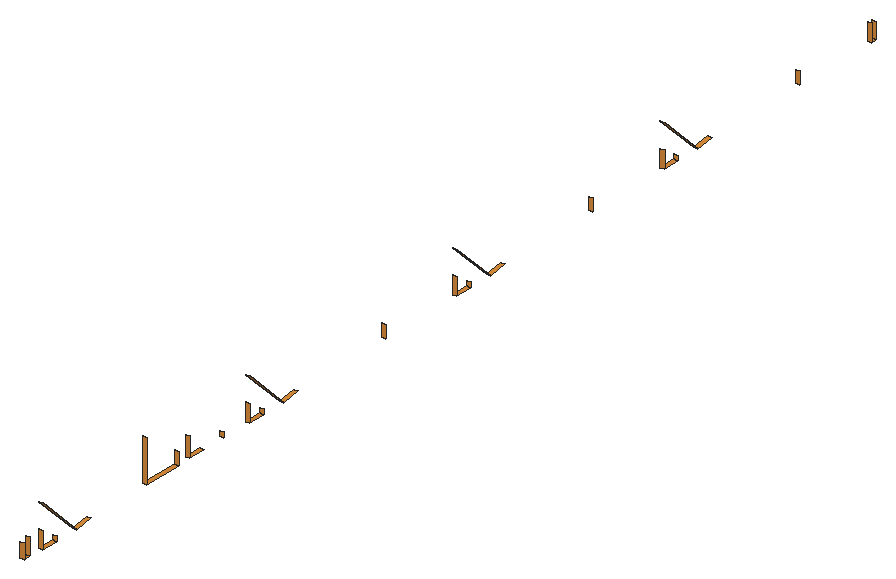
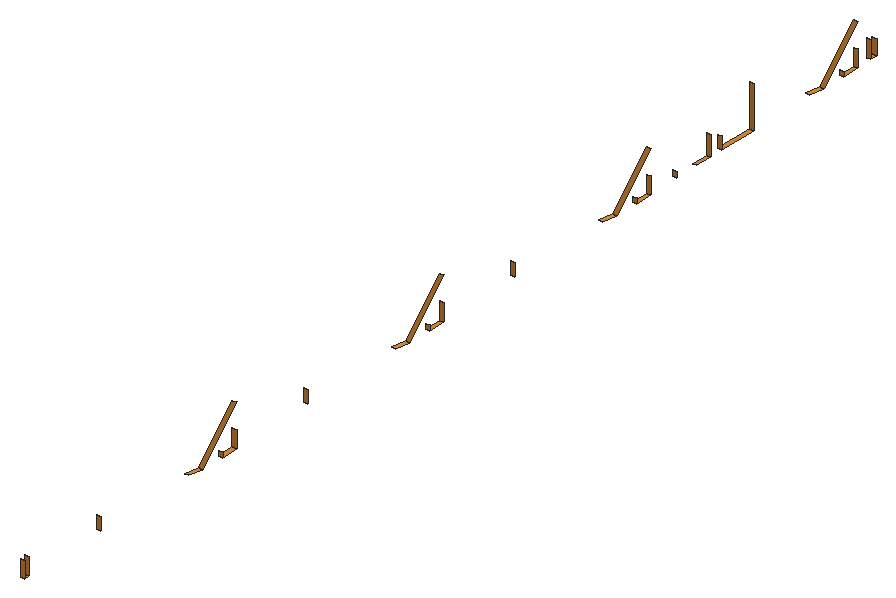
# SketchUp Ruby script. Lengths in inches.
U = 1.inch
M = Sketchup.active_model
def pt(a) = Geom::Point3d.new(a.map { |v| v * U })
def face(e, loops, mat)
  f = e.add_face(loops[0].map { |a| pt(a) })
  loops[1..].each { |l| e.add_face(l.map { |a| pt(a) }).erase! }
  f.material = f.back_material = mat if mat
  f
end
# faces: each face lists its corners as indices into pts; further lists are holes
def faces(e, pts, list, mat = nil) = list.each { |f| face(e, (f[0].is_a?(Array) ? f : [f]).map { |l| l.map { |i| pts[i] } }, mat) }
# xy, xz, yz: faces in a plane at the given z, y or x. An outline is a flat list of corners, or four numbers for a rectangle; further outlines are holes
def ring(l) = l.size == 4 ? [[l[0], l[1]], [l[2], l[1]], [l[2], l[3]], [l[0], l[3]]] : l.each_slice(2).to_a
def flat(e, list, mat, &to3) = list.each { |f| face(e, (f[0].is_a?(Array) ? f : [f]).map { |l| ring(l).map { |u, v| to3.(u, v) } }, mat) }
def xy(e, z, list, mat = nil) = flat(e, list, mat) { |x, y| [x, y, z] }
def xz(e, y, list, mat = nil) = flat(e, list, mat) { |x, z| [x, y, z] }
def yz(e, x, list, mat = nil) = flat(e, list, mat) { |y, z| [x, y, z] }
def lines(e, pts, list) = list.each { |a, b| e.add_line(pt(pts[a]), pt(pts[b])) }
# prism: a flat outline (further loops are holes) pulled along v
def prism(e, loops, v, mat = nil)
  f = face(e, loops, mat); d = Geom::Vector3d.new(v.map { |x| x * U })
  f.pushpull(f.normal.samedirection?(d) ? d.length : -d.length)
end
def box(e, o, s, mat = nil) = prism(e, [[o, [o[0] + s[0], o[1], o[2]], [o[0] + s[0], o[1] + s[1], o[2]], [o[0], o[1] + s[1], o[2]]]], [0, 0, s[2]], mat)
def at(x, y, z, deg = 0) = Geom::Transformation.translation(pt([x, y, z])) * Geom::Transformation.rotation(ORIGIN, Z_AXIS, deg.degrees)
def axes(o, x, y, z) = Geom::Transformation.new([*x, 0, *y, 0, *z, 0, *pt(o).to_a, 1])
def part(name) = M.definitions.add(name)
# library, detail: a bought-in or finely detailed component or shape, given as its bounding box
def library(name, o, s) = part(name).tap { |d| box(d.entities, o, s) }
def detail(e, o, s) = box(e.add_group.entities, o, s)
def put(e, d, t, mat = nil) = e.add_instance(d, t).tap { |i| i.material = mat if mat }
def group(e, t, mat = nil) = e.add_group.tap { |g| g.transformation = t; g.material = mat if mat }.entities
root = M.entities
M.materials.add("1056 AP 9903 Mellow Melon-N").color = [219, 142, 59]
xy(root,148.04,[[14.35,18.88,15.0625,21.91],[14.35,64.22,15.0625,67.26],[14.35,109.57,15.0625,112.6],[14.35,154.91,15.0625,157.94],[14.35,200.25,15.0625,201.3125]],"1056 AP 9903 Mellow Melon-N")
xy(root,148.27,[[14.35,14.79,15.0625,16.07],[14.35,41.65,15.0625,48.53],[14.35,51.11,15.0625,54.08]],"1056 AP 9903 Mellow Melon-N")
xz(root,14.79,[[14.35,148.27,15.0625,150.86]],"1056 AP 9903 Mellow Melon-N")
xz(root,16.07,[[14.35,148.27,15.0625,151.3]],"1056 AP 9903 Mellow Melon-N")
xz(root,18.88,[[14.35,148.04,15.0625,151.05]],"1056 AP 9903 Mellow Melon-N")
xz(root,21.91,[[14.35,148.04,15.0625,148.89]],"1056 AP 9903 Mellow Melon-N")
xz(root,41.65,[[14.35,148.27,15.0625,155.63]],"1056 AP 9903 Mellow Melon-N")
xz(root,48.53,[[14.35,148.27,15.0625,150.43]],"1056 AP 9903 Mellow Melon-N")
xz(root,51.11,[[14.35,148.27,15.0625,151.76]],"1056 AP 9903 Mellow Melon-N")
xz(root,58.41,[[14.35,148.27,15.0625,149.14]],"1056 AP 9903 Mellow Melon-N")
xz(root,64.22,[[14.35,148.04,15.0625,151.05]],"1056 AP 9903 Mellow Melon-N")
xz(root,67.26,[[14.35,148.04,15.0625,148.89]],"1056 AP 9903 Mellow Melon-N")
xz(root,93.87,[[14.35,148.27,15.0625,150.43]],"1056 AP 9903 Mellow Melon-N")
xz(root,109.57,[[14.35,148.04,15.0625,151.05]],"1056 AP 9903 Mellow Melon-N")
xz(root,112.6,[[14.35,148.04,15.0625,148.89]],"1056 AP 9903 Mellow Melon-N")
xz(root,139.21,[[14.35,148.27,15.0625,150.43]],"1056 AP 9903 Mellow Melon-N")
xz(root,154.91,[[14.35,148.04,15.0625,151.05]],"1056 AP 9903 Mellow Melon-N")
xz(root,157.94,[[14.35,148.04,15.0625,148.89]],"1056 AP 9903 Mellow Melon-N")
xz(root,184.56,[[14.35,148.27,15.0625,150.43]],"1056 AP 9903 Mellow Melon-N")
xz(root,200.25,[[14.35,148.04,15.0625,151.05]],"1056 AP 9903 Mellow Melon-N")
xz(root,201.3125,[[14.35,148.04,15.0625,150.86]],"1056 AP 9903 Mellow Melon-N")
p = [[15.0625,18.88,155.375],[15.0625,26.22,148.03],[14.35,26.22,148.03],[14.35,18.88,155.375],[15.0625,29.28,148.47],[14.35,29.28,148.47],
  [15.0625,64.22,155.375],[15.0625,71.5625,148.03],[14.35,71.5625,148.03],[14.35,64.22,155.375],[15.0625,74.625,148.47],[14.35,74.625,148.47],
  [15.0625,109.57,155.375],[15.0625,116.91,148.03],[14.35,116.91,148.03],[14.35,109.57,155.375],[15.0625,119.97,148.47],[14.35,119.97,148.47],
  [15.0625,154.91,155.375],[15.0625,162.25,148.03],[14.35,162.25,148.03],[14.35,154.91,155.375],[15.0625,165.3125,148.47],[14.35,165.3125,148.47]]
faces(root,p,[[0,1,2,3],[1,4,5,2],[6,7,8,9],[7,10,11,8],[12,13,14,15],[13,16,17,14],[18,19,20,21],[19,22,23,20]],"1056 AP 9903 Mellow Melon-N")
